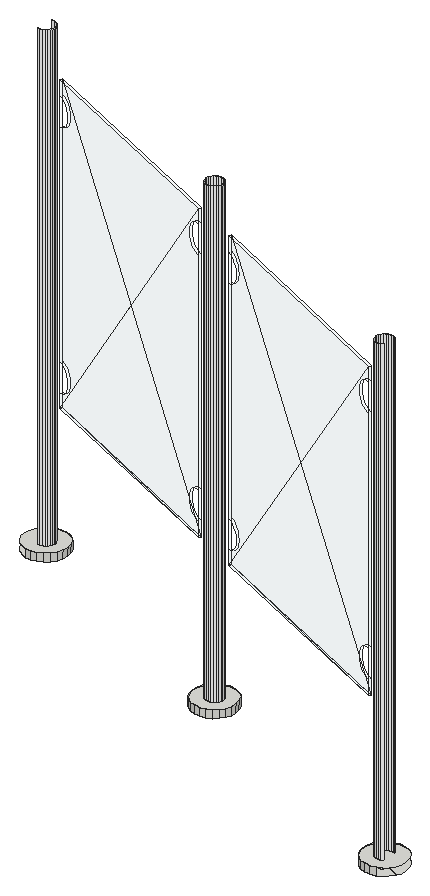
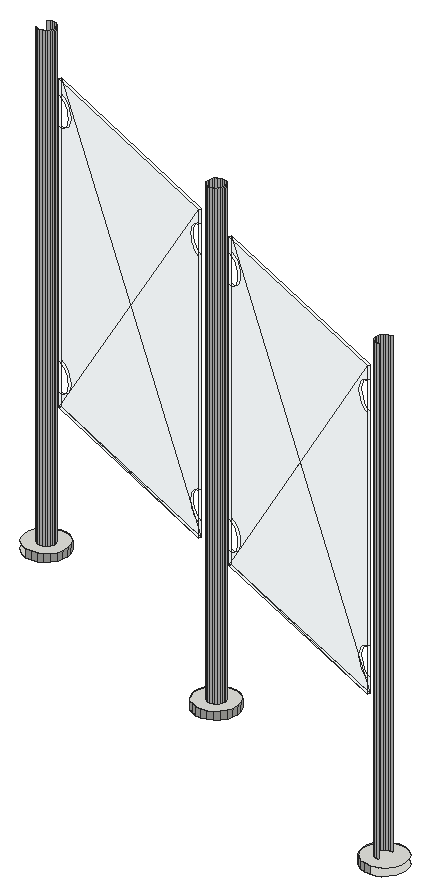
# SketchUp Ruby script. Lengths in inches.
U = 1.inch
M = Sketchup.active_model
def pt(a) = Geom::Point3d.new(a.map { |v| v * U })
def face(e, loops, mat)
  f = e.add_face(loops[0].map { |a| pt(a) })
  loops[1..].each { |l| e.add_face(l.map { |a| pt(a) }).erase! }
  f.material = f.back_material = mat if mat
  f
end
# faces: each face lists its corners as indices into pts; further lists are holes
def faces(e, pts, list, mat = nil) = list.each { |f| face(e, (f[0].is_a?(Array) ? f : [f]).map { |l| l.map { |i| pts[i] } }, mat) }
# xy, xz, yz: faces in a plane at the given z, y or x. An outline is a flat list of corners, or four numbers for a rectangle; further outlines are holes
def ring(l) = l.size == 4 ? [[l[0], l[1]], [l[2], l[1]], [l[2], l[3]], [l[0], l[3]]] : l.each_slice(2).to_a
def flat(e, list, mat, &to3) = list.each { |f| face(e, (f[0].is_a?(Array) ? f : [f]).map { |l| ring(l).map { |u, v| to3.(u, v) } }, mat) }
def xy(e, z, list, mat = nil) = flat(e, list, mat) { |x, y| [x, y, z] }
def xz(e, y, list, mat = nil) = flat(e, list, mat) { |x, z| [x, y, z] }
def yz(e, x, list, mat = nil) = flat(e, list, mat) { |y, z| [x, y, z] }
def lines(e, pts, list) = list.each { |a, b| e.add_line(pt(pts[a]), pt(pts[b])) }
# prism: a flat outline (further loops are holes) pulled along v
def prism(e, loops, v, mat = nil)
  f = face(e, loops, mat); d = Geom::Vector3d.new(v.map { |x| x * U })
  f.pushpull(f.normal.samedirection?(d) ? d.length : -d.length)
end
def box(e, o, s, mat = nil) = prism(e, [[o, [o[0] + s[0], o[1], o[2]], [o[0] + s[0], o[1] + s[1], o[2]], [o[0], o[1] + s[1], o[2]]]], [0, 0, s[2]], mat)
def at(x, y, z, deg = 0) = Geom::Transformation.translation(pt([x, y, z])) * Geom::Transformation.rotation(ORIGIN, Z_AXIS, deg.degrees)
def axes(o, x, y, z) = Geom::Transformation.new([*x, 0, *y, 0, *z, 0, *pt(o).to_a, 1])
def part(name) = M.definitions.add(name)
# library, detail: a bought-in or finely detailed component or shape, given as its bounding box
def library(name, o, s) = part(name).tap { |d| box(d.entities, o, s) }
def detail(e, o, s) = box(e.add_group.entities, o, s)
def put(e, d, t, mat = nil) = e.add_instance(d, t).tap { |i| i.material = mat if mat }
def group(e, t, mat = nil) = e.add_group.tap { |g| g.transformation = t; g.material = mat if mat }.entities
root = M.entities
M.materials.add("Glass_Safety_01").color = [204, 235, 244]
M.materials["Glass_Safety_01"].alpha = 0.1
M.materials.add("[Color_000]").color = [255, 255, 255]
xy(root,321.27,[[[612.53,632.98,612.9375,633.0625,613.3,633.25,613.61,633.52,613.84,633.86,613.97,634.25,613.99,634.66,613.91,635.06,613.73,635.43,613.45,635.74,613.11,635.97,612.72,636.1,612.31,636.12,611.91,636.04,611.54,635.85,611.23,635.58,611,635.24,610.98,635.18,610.875,634.85,610.85,634.4375,610.93,634.03,611.12,633.67,611.39,633.36,611.73,633.13,612.125,633],[612.47,633.92,612.3,633.93,612.15,633.98,612.01,634.07,611.9,634.2,611.83,634.34,611.79,634.5,611.8,634.67,611.85,634.8,611.85,634.82,611.95,634.96,612.07,635.07,612.22,635.14,612.375,635.18,612.54,635.17,612.7,635.12,612.83,635.03,612.94,634.9,613.02,634.76,613.05,634.59,613.04,634.43,613,634.3,612.99,634.27,612.9,634.14,612.77,634.03,612.63,633.95]],[613.86,633.92,613.97,634.25,613.99,634.66,613.91,635.06,613.73,635.43,613.45,635.74,613.11,635.97,612.72,636.1,612.31,636.12,611.91,636.04,611.54,635.85,611.23,635.58,611,635.24,610.98,635.18,611.85,634.8,611.85,634.82,611.95,634.96,612.07,635.07,612.22,635.14,612.375,635.18,612.54,635.17,612.7,635.12,612.83,635.03,612.94,634.9,613.02,634.76,613.05,634.59,613.04,634.43,613,634.3],[613,634.3,613.04,634.43,613.05,634.59,613.02,634.76,612.94,634.9,612.83,635.03,612.7,635.12,612.54,635.17,612.375,635.18,612.22,635.14,612.07,635.07,611.95,634.96,611.85,634.82,611.85,634.8],[[592.54,641.6875,592.94,641.77,593.31,641.95,593.62,642.23,593.84,642.57,593.97,642.96,594,643.37,593.91,643.77,593.73,644.14,593.46,644.45,593.11,644.67,592.72,644.8,592.3125,644.83,591.91,644.75,591.54,644.5625,591.24,644.29,591.01,643.95,590.99,643.88,590.88,643.56,590.85,643.15,590.9375,642.74,591.12,642.375,591.39,642.07,591.74,641.84,592.13,641.71],[592.47,642.63,592.31,642.64,592.15,642.69,592.01,642.78,591.9,642.91,591.83,643.05,591.8,643.21,591.81,643.38,591.85,643.51,591.86,643.53,591.95,643.67,592.07,643.78,592.22,643.85,592.38,643.89,592.54,643.875,592.7,643.83,592.84,643.73,592.95,643.61,593.02,643.46,593.05,643.3,593.04,643.14,593,643.01,592.99,642.98,592.9,642.85,592.78,642.74,592.63,642.66]],[593.86,642.63,593.97,642.96,594,643.37,593.91,643.77,593.73,644.14,593.46,644.45,593.11,644.67,592.72,644.8,592.3125,644.83,591.91,644.75,591.54,644.5625,591.24,644.29,591.01,643.95,590.99,643.88,591.85,643.51,591.86,643.53,591.95,643.67,592.07,643.78,592.22,643.85,592.38,643.89,592.54,643.875,592.7,643.83,592.84,643.73,592.95,643.61,593.02,643.46,593.05,643.3,593.04,643.14,593,643.01],
  [593,643.01,593.04,643.14,593.05,643.3,593.02,643.46,592.95,643.61,592.84,643.73,592.7,643.83,592.54,643.875,592.38,643.89,592.22,643.85,592.07,643.78,591.95,643.67,591.86,643.53,591.85,643.51],[[572.73,650.32,573.13,650.4,573.5,650.58,573.8,650.86,574.03,651.2,574.16,651.59,574.18,652,574.1,652.4,573.92,652.77,573.64,653.08,573.3,653.3,572.91,653.43,572.5,653.46,572.1,653.375,571.73,653.19,571.42,652.92,571.2,652.58,571.18,652.51,571.07,652.18,571.04,651.77,571.125,651.37,571.31,651,571.58,650.7,571.93,650.47,572.32,650.34],[572.66,651.26,572.49,651.27,572.34,651.32,572.2,651.41,572.09,651.53,572.02,651.68,571.99,651.84,571.99,652.01,572.04,652.14,572.05,652.16,572.14,652.3,572.26,652.41,572.41,652.48,572.57,652.52,572.73,652.51,572.89,652.45,573.03,652.36,573.13,652.24,573.21,652.09,573.24,651.93,573.23,651.77,573.1875,651.64,573.18,651.61,573.09,651.47,572.97,651.37,572.82,651.29]],[574.05,651.26,574.16,651.59,574.18,652,574.1,652.4,573.92,652.77,573.64,653.08,573.3,653.3,572.91,653.43,572.5,653.46,572.1,653.375,571.73,653.19,571.42,652.92,571.2,652.58,571.18,652.51,572.04,652.14,572.05,652.16,572.14,652.3,572.26,652.41,572.41,652.48,572.57,652.52,572.73,652.51,572.89,652.45,573.03,652.36,573.13,652.24,573.21,652.09,573.24,651.93,573.23,651.77,573.1875,651.64],[573.1875,651.64,573.23,651.77,573.24,651.93,573.21,652.09,573.13,652.24,573.03,652.36,572.89,652.45,572.73,652.51,572.57,652.52,572.41,652.48,572.26,652.41,572.14,652.3,572.05,652.16,572.04,652.14]])
xy(root,321.27,[[612.47,633.92,612.63,633.95,612.77,634.03,612.9,634.14,612.99,634.27,613,634.3,611.85,634.8,611.8,634.67,611.79,634.5,611.83,634.34,611.9,634.2,612.01,634.07,612.15,633.98,612.3,633.93],[592.47,642.63,592.63,642.66,592.78,642.74,592.9,642.85,592.99,642.98,593,643.01,591.85,643.51,591.81,643.38,591.8,643.21,591.83,643.05,591.9,642.91,592.01,642.78,592.15,642.69,592.31,642.64]],"[Color_000]")
xy(root,321.86,[[612.53,632.98,612.9375,633.0625,613.3,633.25,613.61,633.52,613.84,633.86,613.97,634.25,613.99,634.66,613.91,635.06,613.73,635.43,613.45,635.74,613.11,635.97,612.72,636.1,612.31,636.12,611.91,636.04,611.54,635.85,611.23,635.58,611,635.24,610.875,634.85,610.85,634.4375,610.93,634.03,611.12,633.67,611.39,633.36,611.73,633.13,612.125,633],[592.54,641.6875,592.94,641.77,593.31,641.95,593.62,642.23,593.84,642.57,593.97,642.96,594,643.37,593.91,643.77,593.73,644.14,593.46,644.45,593.11,644.67,592.72,644.8,592.3125,644.83,591.91,644.75,591.54,644.5625,591.24,644.29,591.01,643.95,590.88,643.56,590.85,643.15,590.9375,642.74,591.12,642.375,591.39,642.07,591.74,641.84,592.13,641.71],[572.73,650.32,573.13,650.4,573.5,650.58,573.8,650.86,574.03,651.2,574.16,651.59,574.18,652,574.1,652.4,573.92,652.77,573.64,653.08,573.3,653.3,572.91,653.43,572.5,653.46,572.1,653.375,571.73,653.19,571.42,652.92,571.2,652.58,571.07,652.18,571.04,651.77,571.125,651.37,571.31,651,571.58,650.7,571.93,650.47,572.32,650.34]])
xy(root,331.9,[[610.74,635.17,594.19,642.38,594.27,642.5625],[610.74,635.17,594.27,642.5625,610.82,635.35],[590.75,643.88,574.38,651.01,574.46,651.19],[590.75,643.88,574.46,651.19,590.82,644.0625]],"Glass_Safety_01")
p = [[611.73,633.13,321.27],[612.125,633,321.27],[612.125,633,321.86],[611.73,633.13,321.86],[612.53,632.98,321.27],[612.53,632.98,321.86],
  [612.9375,633.0625,321.27],[612.9375,633.0625,321.86],[611.39,633.36,321.27],[611.39,633.36,321.86],[611.12,633.67,321.27],[611.12,633.67,321.86],
  [610.93,634.03,321.27],[610.93,634.03,321.86],[612.15,633.98,321.27],[612.3,633.93,321.27],[612.3,633.93,357.27],[612.15,633.98,357.27],
  [612.47,633.92,321.27],[612.47,633.92,357.27],[612.63,633.95,321.27],[612.63,633.95,357.27],[610.85,634.4375,321.27],[610.85,634.4375,321.86],
  [612.01,634.07,321.27],[612.01,634.07,357.27],[612.77,634.03,321.27],[612.77,634.03,357.27],[611.9,634.2,321.27],[611.9,634.2,357.27],
  [611.83,634.34,321.27],[611.83,634.34,357.27],[611.79,634.5,321.27],[611.79,634.5,357.27],[610.875,634.85,321.27],[610.875,634.85,321.86],
  [611.8,634.67,321.27],[611.8,634.67,357.27],[611.85,634.82,321.27],[611.85,634.8,321.27],[611.85,634.82,357.27],[611,635.24,321.27],
  [610.98,635.18,321.27],[611,635.24,321.86],[611.95,634.96,321.27],[611.95,634.96,357.27],[612.07,635.07,321.27],[612.07,635.07,357.27],
  [612.83,635.03,321.27],[612.7,635.12,321.27],[612.7,635.12,357.27],[612.83,635.03,357.27],[612.22,635.14,321.27],[612.22,635.14,357.27],
  [612.375,635.18,321.27],[612.375,635.18,357.27],[612.54,635.17,321.27],[612.54,635.17,357.27],[611.23,635.58,321.27],[611.23,635.58,321.86],
  [611.54,635.85,321.27],[611.54,635.85,321.86],[611.91,636.04,321.27],[611.91,636.04,321.86],[612.31,636.12,321.27],[612.31,636.12,321.86],
  [612.72,636.1,321.27],[612.72,636.1,321.86],[591.74,641.84,321.27],[592.13,641.71,321.27],[592.13,641.71,321.86],[591.74,641.84,321.86],
  [592.54,641.6875,321.27],[592.54,641.6875,321.86],[592.94,641.77,321.27],[592.94,641.77,321.86],[591.39,642.07,321.27],[591.39,642.07,321.86],
  [593.31,641.95,321.27],[593.31,641.95,321.86],[593.62,642.23,321.27],[593.62,642.23,321.86],[591.12,642.375,321.27],[591.12,642.375,321.86],
  [593.84,642.57,321.27],[593.84,642.57,321.86],[590.9375,642.74,321.27],[590.9375,642.74,321.86],[592.15,642.69,321.27],[592.31,642.64,321.27],
  [592.31,642.64,357.27],[592.15,642.69,357.27],[592.47,642.63,321.27],[592.47,642.63,357.27],[592.63,642.66,321.27],[592.63,642.66,357.27],
  [593.86,642.63,321.27],[593.97,642.96,321.27],[593.97,642.96,321.86],[590.85,643.15,321.27],[590.85,643.15,321.86],[592.01,642.78,321.27],
  [592.01,642.78,357.27],[592.78,642.74,321.27],[592.78,642.74,357.27],[592.9,642.85,321.27],[592.9,642.85,357.27],[591.9,642.91,321.27],
  [591.9,642.91,357.27],[592.99,642.98,321.27],[592.99,642.98,357.27],[591.83,643.05,321.27],[591.83,643.05,357.27],[593,643.01,321.27],
  [593.04,643.14,321.27],[593.04,643.14,357.27],[594,643.37,321.27],[594,643.37,321.86],[590.88,643.56,321.27],[590.88,643.56,321.86],
  [591.8,643.21,321.27],[591.8,643.21,357.27],[593.05,643.3,321.27],[593.05,643.3,357.27],[591.81,643.38,321.27],[591.81,643.38,357.27],
  [593.02,643.46,321.27],[593.02,643.46,357.27],[591.86,643.53,321.27],[591.85,643.51,321.27],[591.86,643.53,357.27],[593.91,643.77,321.27],
  [593.91,643.77,321.86],[591.95,643.67,321.27],[591.95,643.67,357.27],[592.95,643.61,321.27],[592.95,643.61,357.27],[591.01,643.95,321.27],
  [590.99,643.88,321.27],[591.01,643.95,321.86],[592.84,643.73,321.27],[592.84,643.73,357.27],[592.07,643.78,321.27],[592.07,643.78,357.27],
  [592.7,643.83,321.27],[592.7,643.83,357.27],[592.22,643.85,321.27],[592.22,643.85,357.27],[592.54,643.875,321.27],[592.54,643.875,357.27],
  [593.73,644.14,321.27],[593.73,644.14,321.86],[591.24,644.29,321.27],[591.24,644.29,321.86],[592.38,643.89,321.27],[592.38,643.89,357.27],
  [593.46,644.45,321.27],[593.46,644.45,321.86],[591.54,644.5625,321.27],[591.54,644.5625,321.86],[593.11,644.67,321.27],[593.11,644.67,321.86],
  [591.91,644.75,321.27],[591.91,644.75,321.86],[592.3125,644.83,321.27],[592.3125,644.83,321.86],[592.72,644.8,321.27],[592.72,644.8,321.86],
  [572.32,650.34,321.27],[572.73,650.32,321.27],[572.73,650.32,321.86],[572.32,650.34,321.86],[573.13,650.4,321.27],[573.13,650.4,321.86],
  [573.5,650.58,321.27],[573.5,650.58,321.86],[573.8,650.86,321.27],[573.8,650.86,321.86],[574.03,651.2,321.27],[574.03,651.2,321.86],
  [574.05,651.26,321.27],[574.16,651.59,321.27],[574.16,651.59,321.86],[572.49,651.27,321.27],[572.66,651.26,321.27],[572.66,651.26,357.27],
  [572.49,651.27,357.27],[572.82,651.29,321.27],[572.82,651.29,357.27],[572.97,651.37,321.27],[572.97,651.37,357.27],[573.09,651.47,321.27],
  [573.09,651.47,357.27],[573.18,651.61,321.27],[573.18,651.61,357.27],[573.1875,651.64,321.27],[573.23,651.77,321.27],[573.23,651.77,357.27],
  [574.18,652,321.27],[574.18,652,321.86],[573.24,651.93,321.27],[573.24,651.93,357.27],[573.21,652.09,321.27],[573.21,652.09,357.27],
  [574.1,652.4,321.27],[574.1,652.4,321.86],[573.13,652.24,321.27],[573.13,652.24,357.27],[573.03,652.36,321.27],[573.03,652.36,357.27],
  [572.89,652.45,321.27],[572.89,652.45,357.27],[573.92,652.77,321.27],[573.92,652.77,321.86],[572.73,652.51,321.27],[572.57,652.52,321.27],
  [572.57,652.52,357.27],[572.73,652.51,357.27],[573.64,653.08,321.27],[573.64,653.08,321.86],[573.3,653.3,321.27],[573.3,653.3,321.86],
  [572.91,653.43,321.27],[572.91,653.43,321.86],[572.5,653.46,321.27],[572.5,653.46,321.86],[594.19,642.38,351.28],[594.19,642.38,335.125],
  [594.44,642.27,335.09],[594.68,642.17,334.98],[594.88,642.08,334.8125],[595.03,642.01,334.59],[595.13,641.97,334.34],[595.17,641.96,334.0625],
  [595.13,641.97,333.79],[595.03,642.01,333.53],[594.88,642.08,333.3125],[594.68,642.17,333.14],[594.44,642.27,333.04],[594.19,642.38,333],
  [594.19,642.38,331.9],[610.74,635.17,354.51],[594.19,642.38,354.51],[594.19,642.38,353.41],[594.44,642.27,353.37],[594.68,642.17,353.27],
  [594.88,642.08,353.1],[595.03,642.01,352.88],[595.13,641.97,352.62],[595.17,641.96,352.35],[595.13,641.97,352.07],[595.03,642.01,351.81],
  [594.88,642.08,351.59],[594.68,642.17,351.43],[594.44,642.27,351.32],[610.74,635.17,331.9],[610.74,635.17,333],[610.58,635.25,333],
  [610.33,635.36,333.04],[610.09,635.46,333.14],[609.89,635.55,333.3125],[609.73,635.61,333.53],[609.64,635.66,333.79],[609.6,635.67,334.0625],
  [609.64,635.66,334.34],[609.73,635.61,334.59],[609.89,635.55,334.8125],[610.09,635.46,334.98],[610.33,635.36,335.09],[610.58,635.25,335.125],
  [610.74,635.17,335.125],[610.74,635.17,351.28],[610.58,635.25,351.28],[610.33,635.36,351.32],[610.09,635.46,351.43],[609.89,635.55,351.59],
  [609.73,635.61,351.81],[609.64,635.66,352.07],[609.6,635.67,352.35],[609.64,635.66,352.62],[609.73,635.61,352.88],[609.89,635.55,353.1],
  [610.09,635.46,353.27],[610.33,635.36,353.37],[610.58,635.25,353.41],[610.74,635.17,353.41],[610.82,635.35,331.9],[610.82,635.35,333],
  [610.82,635.35,335.125],[610.82,635.35,351.28],[610.82,635.35,353.41],[610.82,635.35,354.51],[594.27,642.5625,331.9],[594.27,642.5625,333],
  [594.52,642.45,333.04],[594.76,642.35,333.14],[594.96,642.26,333.3125],[595.11,642.19,333.53],[595.21,642.15,333.79],[595.24,642.14,334.0625],
  [595.21,642.15,334.34],[595.11,642.19,334.59],[594.96,642.26,334.8125],[594.76,642.35,334.98],[594.52,642.45,335.09],[594.27,642.5625,335.125],
  [594.27,642.5625,351.28],[594.52,642.45,351.32],[594.76,642.35,351.43],[594.96,642.26,351.59],[595.11,642.19,351.81],[595.21,642.15,352.07],
  [595.24,642.14,352.35],[595.21,642.15,352.62],[595.11,642.19,352.88],[594.96,642.26,353.1],[594.76,642.35,353.27],[594.52,642.45,353.37],
  [594.27,642.5625,353.41],[594.27,642.5625,354.51],[610.66,635.43,335.125],[610.4,635.54,335.09],[610.17,635.64,334.98],[609.97,635.73,334.8125],
  [609.8125,635.79,334.59],[609.71,635.84,334.34],[609.68,635.85,334.0625],[609.71,635.84,333.79],[609.8125,635.79,333.53],[609.97,635.73,333.3125],
  [610.17,635.64,333.14],[610.4,635.54,333.04],[610.66,635.43,333],[610.66,635.43,353.41],[610.4,635.54,353.37],[610.17,635.64,353.27],
  [609.97,635.73,353.1],[609.8125,635.79,352.88],[609.71,635.84,352.62],[609.68,635.85,352.35],[609.71,635.84,352.07],[609.8125,635.79,351.81],
  [609.97,635.73,351.59],[610.17,635.64,351.43],[610.4,635.54,351.32],[610.66,635.43,351.28],[574.38,651.01,351.28],[574.38,651.01,335.125],
  [574.63,650.9,335.09],[574.87,650.8,334.98],[575.07,650.71,334.8125],[575.22,650.64,334.59],[575.32,650.6,334.34],[575.35,650.59,334.0625],
  [575.32,650.6,333.79],[575.22,650.64,333.53],[575.07,650.71,333.3125],[574.87,650.8,333.14],[574.63,650.9,333.04],[574.38,651.01,333],
  [574.38,651.01,331.9],[590.75,643.88,354.51],[574.38,651.01,354.51],[574.38,651.01,353.41],[574.63,650.9,353.37],[574.87,650.8,353.27],
  [575.07,650.71,353.1],[575.22,650.64,352.88],[575.32,650.6,352.62],[575.35,650.59,352.35],[575.32,650.6,352.07],[575.22,650.64,351.81],
  [575.07,650.71,351.59],[574.87,650.8,351.43],[574.63,650.9,351.32],[590.75,643.88,331.9],[590.75,643.88,333],[590.58,643.95,333],
  [590.33,644.0625,333.04],[590.09,644.17,333.14],[589.89,644.25,333.3125],[589.74,644.32,333.53],[589.64,644.36,333.79],[589.61,644.38,334.0625],
  [589.64,644.36,334.34],[589.74,644.32,334.59],[589.89,644.25,334.8125],[590.09,644.17,334.98],[590.33,644.0625,335.09],[590.58,643.95,335.125],
  [590.75,643.88,335.125],[590.75,643.88,351.28],[590.58,643.95,351.28],[590.33,644.0625,351.32],[590.09,644.17,351.43],[589.89,644.25,351.59],
  [589.74,644.32,351.81],[589.64,644.36,352.07],[589.61,644.38,352.35],[589.64,644.36,352.62],[589.74,644.32,352.88],[589.89,644.25,353.1],
  [590.09,644.17,353.27],[590.33,644.0625,353.37],[590.58,643.95,353.41],[590.75,643.88,353.41],[590.82,644.0625,331.9],[590.82,644.0625,333],
  [590.82,644.0625,335.125],[590.82,644.0625,351.28],[590.82,644.0625,353.41],[590.82,644.0625,354.51],[574.46,651.19,331.9],[574.46,651.19,333],
  [574.71,651.08,333.04],[574.94,650.98,333.14],[575.15,650.89,333.3125],[575.3,650.82,333.53],[575.4,650.78,333.79],[575.43,650.77,334.0625],
  [575.4,650.78,334.34],[575.3,650.82,334.59],[575.15,650.89,334.8125],[574.94,650.98,334.98],[574.71,651.08,335.09],[574.46,651.19,335.125],
  [574.46,651.19,351.28],[574.71,651.08,351.32],[574.94,650.98,351.43],[575.15,650.89,351.59],[575.3,650.82,351.81],[575.4,650.78,352.07],
  [575.43,650.77,352.35],[575.4,650.78,352.62],[575.3,650.82,352.88],[575.15,650.89,353.1],[574.94,650.98,353.27],[574.71,651.08,353.37],
  [574.46,651.19,353.41],[574.46,651.19,354.51],[590.66,644.13,335.125],[590.41,644.24,335.09],[590.17,644.35,334.98],[589.97,644.43,334.8125],
  [589.82,644.5,334.59],[589.72,644.54,334.34],[589.69,644.56,334.0625],[589.72,644.54,333.79],[589.82,644.5,333.53],[589.97,644.43,333.3125],
  [590.17,644.35,333.14],[590.41,644.24,333.04],[590.66,644.13,333],[590.66,644.13,353.41],[590.41,644.24,353.37],[590.17,644.35,353.27],
  [589.97,644.43,353.1],[589.82,644.5,352.88],[589.72,644.54,352.62],[589.69,644.56,352.35],[589.72,644.54,352.07],[589.82,644.5,351.81],
  [589.97,644.43,351.59],[590.17,644.35,351.43],[590.41,644.24,351.32],[590.66,644.13,351.28]]
faces(root,p,[[0,1,2,3],[1,4,5,2],[4,6,7,5],[8,0,3,9],[10,8,9,11],[12,10,11,13],[22,12,13,23],[34,22,23,35],
  [41,42,34,35,43],[58,41,43,59],[60,58,59,61],[62,60,61,63],[64,62,63,65],[66,64,65,67],[68,69,70,71],[69,72,73,70],
  [72,74,75,73],[76,68,71,77],[74,78,79,75],[78,80,81,79],[82,76,77,83],[80,84,85,81],[86,82,83,87],[84,96,97,98,85],
  [99,86,87,100],[97,116,117,98],[118,99,100,119],[116,131,132,117],[137,138,118,119,139],[131,150,151,132],[152,137,139,153],[150,156,157,151],
  [158,152,153,159],[156,160,161,157],[162,158,159,163],[164,162,163,165],[160,166,167,161],[166,164,165,167],[168,169,170,171],[169,172,173,170],
  [172,174,175,173],[174,176,177,175],[176,178,179,177],[178,180,181,182,179],[181,198,199,182],[198,204,205,199],[204,212,213,205],[212,218,219,213],
  [218,220,221,219],[220,222,223,221],[222,224,225,223]])
faces(root,p,[[14,15,16,17],[15,18,19,16],[18,20,21,19],[24,14,17,25],[20,26,27,21],[28,24,25,29],[30,28,29,31],[32,30,31,33],
  [36,32,33,37],[38,39,36,37,40],[44,38,40,45],[46,44,45,47],[48,49,50,51],[52,46,47,53],[54,52,53,55],[49,56,57,50],
  [56,54,55,57],[88,89,90,91],[89,92,93,90],[92,94,95,93],[101,88,91,102],[94,103,104,95],[103,105,106,104],[107,101,102,108],
  [105,109,110,106],[111,107,108,112],[109,113,114,115,110],[120,111,112,121],[114,122,123,115],[124,120,121,125],[122,126,127,123],[128,129,124,125,130],
  [133,128,130,134],[126,135,136,127],[135,140,141,136],[142,133,134,143],[140,144,145,141],[146,142,143,147],[144,148,149,145],[154,146,147,155],
  [148,154,155,149],[183,184,185,186],[184,187,188,185],[187,189,190,188],[189,191,192,190],[191,193,194,192],[193,195,196,197,194],[196,200,201,197],
  [200,202,203,201],[202,206,207,203],[206,208,209,207],[208,210,211,209],[214,215,216,217],[210,214,217,211]],"[Color_000]")
faces(root,p,[[226,227,228,229,230,231,232,233,234,235,236,237,238,239,240,241,242,243,244,245,246,247,248,249,250,251,252,253,254],[255,256,257,258,259,260,261,262,263,264,265,266,267,268,269,270,271,272,273,274,275,276,277,278,279,280,281,282,283,284,285,241,240],[255,286,287,288,289,290,291,241,285,271,270,256],[292,293,294,295,296,297,298,299,300,301,302,303,304,305,306,307,308,309,310,311,312,313,314,315,316,317,318,319,286],[289,288,320,321,322,323,324,325,326,327,328,329,330,331,332,287,286,319,291,290,333,334,335,336,337,338,339,340,341,342,343,344,345],[292,240,239,227,226,243,242,319,318,306,305,293],[346,347,348,349,350,351,352,353,354,355,356,357,358,359,360,361,362,363,364,365,366,367,368,369,370,371,372,373,374],[375,376,377,378,379,380,381,382,383,384,385,386,387,388,389,390,391,392,393,394,395,396,397,398,399,400,401,402,403,404,405,361,360],
  [375,406,407,408,409,410,411,361,405,391,390,376],[412,413,414,415,416,417,418,419,420,421,422,423,424,425,426,427,428,429,430,431,432,433,434,435,436,437,438,439,406],[409,408,440,441,442,443,444,445,446,447,448,449,450,451,452,407,406,439,411,410,453,454,455,456,457,458,459,460,461,462,463,464,465],[412,360,359,347,346,363,362,439,438,426,425,413]],"Glass_Safety_01")
